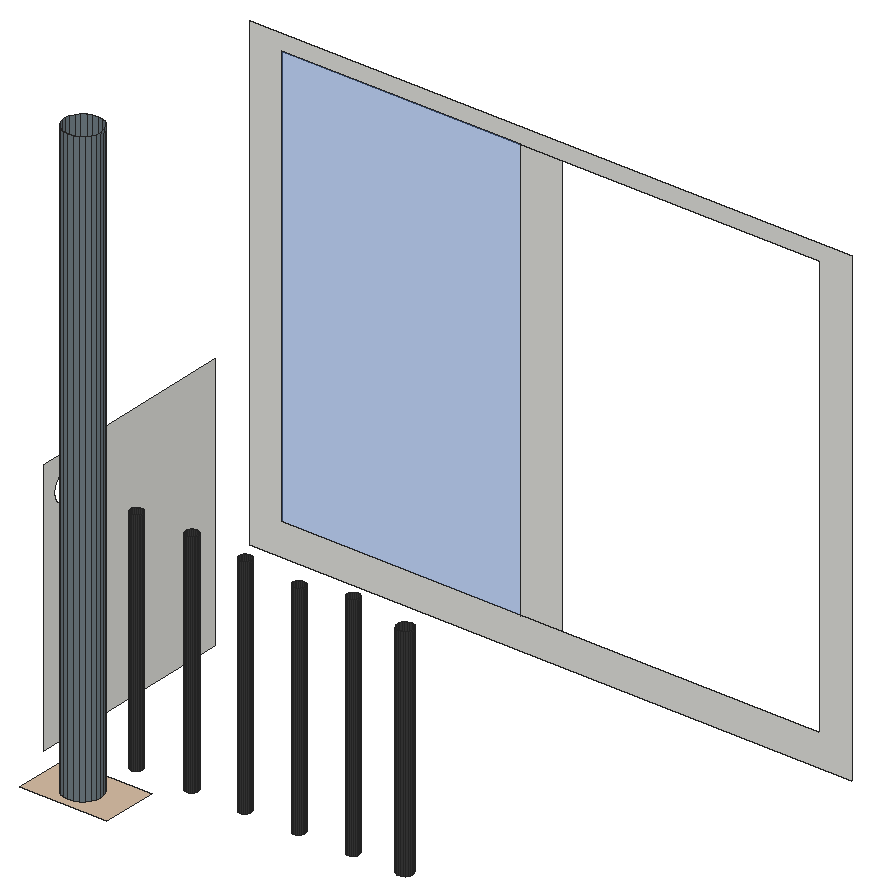
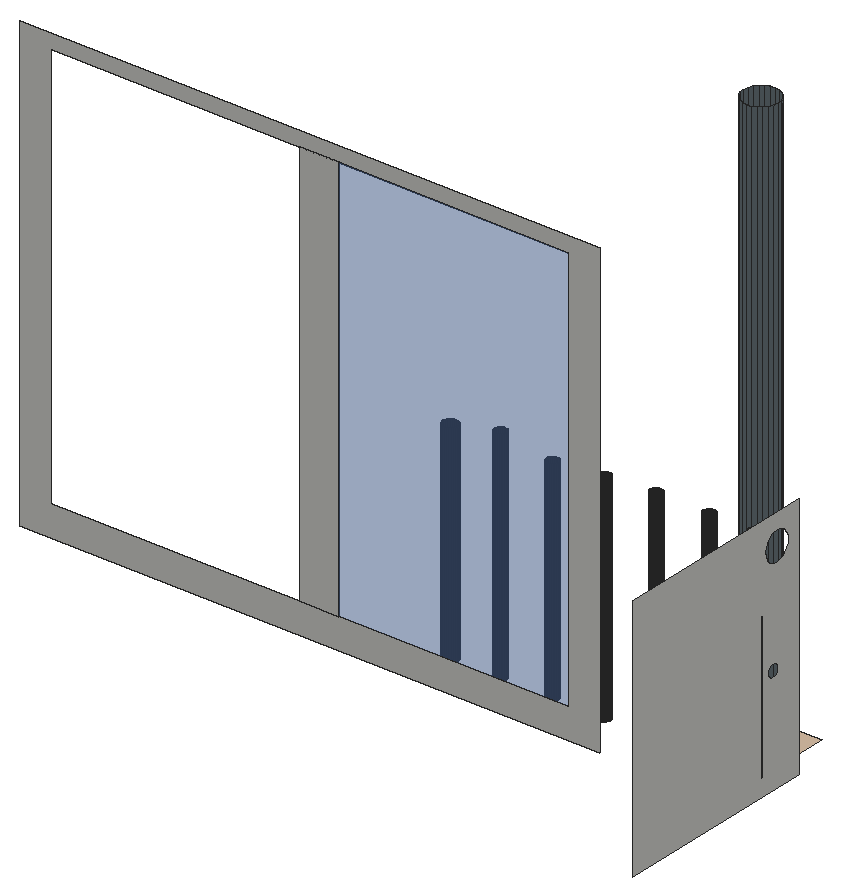
# SketchUp Ruby script. Lengths in inches.
U = 1.inch
M = Sketchup.active_model
def pt(a) = Geom::Point3d.new(a.map { |v| v * U })
def face(e, loops, mat)
  f = e.add_face(loops[0].map { |a| pt(a) })
  loops[1..].each { |l| e.add_face(l.map { |a| pt(a) }).erase! }
  f.material = f.back_material = mat if mat
  f
end
# faces: each face lists its corners as indices into pts; further lists are holes
def faces(e, pts, list, mat = nil) = list.each { |f| face(e, (f[0].is_a?(Array) ? f : [f]).map { |l| l.map { |i| pts[i] } }, mat) }
# xy, xz, yz: faces in a plane at the given z, y or x. An outline is a flat list of corners, or four numbers for a rectangle; further outlines are holes
def ring(l) = l.size == 4 ? [[l[0], l[1]], [l[2], l[1]], [l[2], l[3]], [l[0], l[3]]] : l.each_slice(2).to_a
def flat(e, list, mat, &to3) = list.each { |f| face(e, (f[0].is_a?(Array) ? f : [f]).map { |l| ring(l).map { |u, v| to3.(u, v) } }, mat) }
def xy(e, z, list, mat = nil) = flat(e, list, mat) { |x, y| [x, y, z] }
def xz(e, y, list, mat = nil) = flat(e, list, mat) { |x, z| [x, y, z] }
def yz(e, x, list, mat = nil) = flat(e, list, mat) { |y, z| [x, y, z] }
def lines(e, pts, list) = list.each { |a, b| e.add_line(pt(pts[a]), pt(pts[b])) }
# prism: a flat outline (further loops are holes) pulled along v
def prism(e, loops, v, mat = nil)
  f = face(e, loops, mat); d = Geom::Vector3d.new(v.map { |x| x * U })
  f.pushpull(f.normal.samedirection?(d) ? d.length : -d.length)
end
def box(e, o, s, mat = nil) = prism(e, [[o, [o[0] + s[0], o[1], o[2]], [o[0] + s[0], o[1] + s[1], o[2]], [o[0], o[1] + s[1], o[2]]]], [0, 0, s[2]], mat)
def at(x, y, z, deg = 0) = Geom::Transformation.translation(pt([x, y, z])) * Geom::Transformation.rotation(ORIGIN, Z_AXIS, deg.degrees)
def axes(o, x, y, z) = Geom::Transformation.new([*x, 0, *y, 0, *z, 0, *pt(o).to_a, 1])
def part(name) = M.definitions.add(name)
# library, detail: a bought-in or finely detailed component or shape, given as its bounding box
def library(name, o, s) = part(name).tap { |d| box(d.entities, o, s) }
def detail(e, o, s) = box(e.add_group.entities, o, s)
def put(e, d, t, mat = nil) = e.add_instance(d, t).tap { |i| i.material = mat if mat }
def group(e, t, mat = nil) = e.add_group.tap { |g| g.transformation = t; g.material = mat if mat }.entities
root = M.entities
M.materials.add("[Color M07]").color = [58, 58, 58]
M.materials.add("[Formica Laminate Light]").color = [213, 189, 164]
M.materials.add("[Formica Speckled Grey]").color = [112, 125, 132]
M.materials.add("[Translucent Glass Blue]").color = [85, 126, 201]
M.materials["[Translucent Glass Blue]"].alpha = 0.5
xy(root,273.71,[[54.33,84.29,53.8,84.36,53.3,84.57,52.875,84.89,52.55,85.32,52.34,85.82,52.27,86.35,52.34,86.89,52.55,87.38,52.875,87.8125,53.3,88.14,53.8,88.35,54.33,88.42,54.87,88.35,55.37,88.14,55.79,87.8125,56.12,87.38,56.33,86.89,56.4,86.35,56.33,85.82,56.12,85.32,55.79,84.89,55.37,84.57,54.87,84.36],[85.8,91.86,85.57,91.89,85.36,91.97,85.18,92.11,85.04,92.29,84.95,92.5,84.92,92.73,84.95,92.96,85.04,93.17,85.18,93.35,85.36,93.49,85.57,93.58,85.8,93.61,86.02,93.58,86.24,93.49,86.42,93.35,86.56,93.17,86.64,92.96,86.67,92.73,86.64,92.5,86.56,92.29,86.42,92.11,86.24,91.97,86.02,91.89],[50.09,91.87,49.91,91.89,49.75,91.96,49.61,92.07,49.5,92.21,49.43,92.38,49.4,92.56,49.43,92.73,49.5,92.9,49.61,93.04,49.75,93.15,49.91,93.22,50.09,93.24,50.27,93.22,50.4375,93.15,50.58,93.04,50.6875,92.9,50.76,92.73,50.78,92.56,50.76,92.38,50.6875,92.21,50.58,92.07,50.4375,91.96,50.27,91.89],[55.47,91.87,55.29,91.89,55.125,91.96,54.98,92.07,54.87,92.21,54.8,92.38,54.78,92.56,54.8,92.73,54.87,92.9,54.98,93.04,55.125,93.15,55.29,93.22,55.47,93.24,55.64,93.22,55.8125,93.15,55.95,93.04,56.0625,92.9,56.13,92.73,56.15,92.56,56.13,92.38,56.0625,92.21,55.95,92.07,55.8125,91.96,55.64,91.89],[61.72,91.87,61.54,91.89,61.375,91.96,61.23,92.07,61.12,92.21,61.05,92.38,61.03,92.56,61.05,92.73,61.12,92.9,61.23,93.04,61.375,93.15,61.54,93.22,61.72,93.24,61.89,93.22,62.0625,93.15,62.2,93.04,62.3125,92.9,62.38,92.73,62.4,92.56,62.38,92.38,62.3125,92.21,62.2,92.07,62.0625,91.96,61.89,91.89],
  [67.78,91.87,67.6,91.89,67.4375,91.96,67.29,92.07,67.18,92.21,67.12,92.38,67.09,92.56,67.12,92.73,67.18,92.9,67.29,93.04,67.4375,93.15,67.6,93.22,67.78,93.24,67.96,93.22,68.125,93.15,68.27,93.04,68.375,92.9,68.44,92.73,68.47,92.56,68.44,92.38,68.375,92.21,68.27,92.07,68.125,91.96,67.96,91.89],[73.9,91.87,73.73,91.89,73.5625,91.96,73.42,92.07,73.31,92.21,73.24,92.38,73.22,92.56,73.24,92.73,73.31,92.9,73.42,93.04,73.5625,93.15,73.73,93.22,73.9,93.24,74.08,93.22,74.25,93.15,74.39,93.04,74.5,92.9,74.57,92.73,74.59,92.56,74.57,92.38,74.5,92.21,74.39,92.07,74.25,91.96,74.08,91.89],[80.03,91.87,79.85,91.89,79.6875,91.96,79.54,92.07,79.43,92.21,79.37,92.38,79.34,92.56,79.37,92.73,79.43,92.9,79.54,93.04,79.6875,93.15,79.85,93.22,80.03,93.24,80.21,93.22,80.375,93.15,80.52,93.04,80.625,92.9,80.69,92.73,80.72,92.56,80.69,92.38,80.625,92.21,80.52,92.07,80.375,91.96,80.21,91.89]])
xy(root,273.71,[[[49.6,83.35,59.49,89.73],[54.33,84.29,53.8,84.36,53.3,84.57,52.875,84.89,52.55,85.32,52.34,85.82,52.27,86.35,52.34,86.89,52.55,87.38,52.875,87.8125,53.3,88.14,53.8,88.35,54.33,88.42,54.87,88.35,55.37,88.14,55.79,87.8125,56.12,87.38,56.33,86.89,56.4,86.35,56.33,85.82,56.12,85.32,55.79,84.89,55.37,84.57,54.87,84.36]]],"[Formica Laminate Light]")
xz(root,114.1,[[[51.12,285.36,119.37,338.67],[54.72,288.95,115.77,336.88]],[81.82,288.95,86.49,336.88]])
xz(root,114.1,[[54.72,288.95,81.82,336.88]],"[Translucent Glass Blue]")
yz(root,47.16,[[[89.73,273.71,114.1,302.83],[92.96,297.54,92.51,297.6,92.09,297.77,91.73,298.05,91.45,298.41,91.27,298.84,91.21,299.29,91.27,299.74,91.45,300.16,91.73,300.53,92.09,300.8,92.51,300.98,92.96,301.04,93.42,300.98,93.84,300.8,94.2,300.53,94.48,300.16,94.65,299.74,94.71,299.29,94.65,298.84,94.48,298.41,94.2,298.05,93.84,297.77,93.42,297.6],[93.52,285.62,93.33,285.64,93.15,285.72,92.99,285.84,92.875,285.99,92.8,286.17,92.77,286.37,92.8,286.5625,92.875,286.74,92.99,286.9,93.15,287.02,93.33,287.09,93.52,287.12,93.72,287.09,93.9,287.02,94.05,286.9,94.17,286.74,94.25,286.5625,94.27,286.37,94.25,286.17,94.17,285.99,94.05,285.84,93.9,285.72,93.72,285.64]]])
p = [[53.8,84.36,273.71],[54.33,84.29,273.71],[54.33,84.29,341.31],[53.8,84.36,341.31],[54.87,84.36,273.71],[54.87,84.36,341.31],
  [53.3,84.57,273.71],[53.3,84.57,341.31],[55.37,84.57,273.71],[55.37,84.57,341.31],[52.875,84.89,273.71],[52.875,84.89,341.31],
  [55.79,84.89,273.71],[55.79,84.89,341.31],[52.55,85.32,273.71],[52.55,85.32,341.31],[56.12,85.32,273.71],[56.12,85.32,341.31],
  [52.34,85.82,273.71],[52.34,85.82,341.31],[56.33,85.82,273.71],[56.33,85.82,341.31],[52.27,86.35,273.71],[52.27,86.35,341.31],
  [56.4,86.35,273.71],[56.4,86.35,341.31],[52.34,86.89,273.71],[52.34,86.89,341.31],[56.33,86.89,273.71],[56.33,86.89,341.31],
  [52.55,87.38,273.71],[52.55,87.38,341.31],[56.12,87.38,273.71],[56.12,87.38,341.31],[52.875,87.8125,273.71],[52.875,87.8125,341.31],
  [55.79,87.8125,273.71],[55.79,87.8125,341.31],[53.3,88.14,273.71],[53.3,88.14,341.31],[55.37,88.14,273.71],[55.37,88.14,341.31],
  [53.8,88.35,273.71],[53.8,88.35,341.31],[54.87,88.35,273.71],[54.87,88.35,341.31],[54.33,88.42,273.71],[54.33,88.42,341.31],
  [49.75,91.96,273.71],[49.91,91.89,273.71],[49.91,91.89,299.71],[49.75,91.96,299.71],[50.09,91.87,273.71],[50.09,91.87,299.71],
  [50.27,91.89,273.71],[50.27,91.89,299.71],[50.4375,91.96,273.71],[50.4375,91.96,299.71],[55.125,91.96,273.71],[55.29,91.89,273.71],
  [55.29,91.89,299.74],[55.125,91.96,299.74],[55.47,91.87,273.71],[55.47,91.87,299.74],[55.64,91.89,273.71],[55.64,91.89,299.74],
  [55.8125,91.96,273.71],[55.8125,91.96,299.74],[61.375,91.96,273.71],[61.54,91.89,273.71],[61.54,91.89,299.74],[61.375,91.96,299.74],
  [61.72,91.87,273.71],[61.72,91.87,299.74],[61.89,91.89,273.71],[61.89,91.89,299.74],[62.0625,91.96,273.71],[62.0625,91.96,299.74],
  [67.4375,91.96,273.71],[67.6,91.89,273.71],[67.6,91.89,299.33],[67.4375,91.96,299.33],[67.78,91.87,273.71],[67.78,91.87,299.33],
  [67.96,91.89,273.71],[67.96,91.89,299.33],[68.125,91.96,273.71],[68.125,91.96,299.33],[73.5625,91.96,273.71],[73.73,91.89,273.71],
  [73.73,91.89,298.77],[73.5625,91.96,298.77],[73.9,91.87,273.71],[73.9,91.87,298.77],[74.08,91.89,273.71],[74.08,91.89,298.77],
  [74.25,91.96,273.71],[74.25,91.96,298.77],[79.6875,91.96,273.71],[79.85,91.89,273.71],[79.85,91.89,299.74],[79.6875,91.96,299.74],
  [80.03,91.87,273.71],[80.03,91.87,299.74],[80.21,91.89,273.71],[80.21,91.89,299.74],[80.375,91.96,273.71],[80.375,91.96,299.74],
  [85.36,91.97,273.71],[85.57,91.89,273.71],[85.57,91.89,298.58],[85.36,91.97,298.58],[85.8,91.86,273.71],[85.8,91.86,298.58],
  [86.02,91.89,273.71],[86.02,91.89,298.58],[86.24,91.97,273.71],[86.24,91.97,298.58],[49.61,92.07,273.71],[49.61,92.07,299.71],
  [50.58,92.07,273.71],[50.58,92.07,299.71],[54.98,92.07,273.71],[54.98,92.07,299.74],[55.95,92.07,273.71],[55.95,92.07,299.74],
  [61.23,92.07,273.71],[61.23,92.07,299.74],[62.2,92.07,273.71],[62.2,92.07,299.74],[67.29,92.07,273.71],[67.29,92.07,299.33],
  [68.27,92.07,273.71],[68.27,92.07,299.33],[73.42,92.07,273.71],[73.42,92.07,298.77],[74.39,92.07,273.71],[74.39,92.07,298.77],
  [79.54,92.07,273.71],[79.54,92.07,299.74],[80.52,92.07,273.71],[80.52,92.07,299.74],[85.18,92.11,273.71],[85.18,92.11,298.58],
  [86.42,92.11,273.71],[86.42,92.11,298.58],[49.5,92.21,273.71],[49.5,92.21,299.71],[50.6875,92.21,273.71],[50.6875,92.21,299.71],
  [54.87,92.21,273.71],[54.87,92.21,299.74],[56.0625,92.21,273.71],[56.0625,92.21,299.74],[61.12,92.21,273.71],[61.12,92.21,299.74],
  [62.3125,92.21,273.71],[62.3125,92.21,299.74],[67.18,92.21,273.71],[67.18,92.21,299.33],[68.375,92.21,273.71],[68.375,92.21,299.33],
  [73.31,92.21,273.71],[73.31,92.21,298.77],[74.5,92.21,273.71],[74.5,92.21,298.77],[79.43,92.21,273.71],[79.43,92.21,299.74],
  [80.625,92.21,273.71],[80.625,92.21,299.74],[85.04,92.29,273.71],[85.04,92.29,298.58],[86.56,92.29,273.71],[86.56,92.29,298.58],
  [49.43,92.38,273.71],[49.43,92.38,299.71],[50.76,92.38,273.71],[50.76,92.38,299.71],[54.8,92.38,273.71],[54.8,92.38,299.74],
  [56.13,92.38,273.71],[56.13,92.38,299.74],[61.05,92.38,273.71],[61.05,92.38,299.74],[62.38,92.38,273.71],[62.38,92.38,299.74],
  [67.12,92.38,273.71],[67.12,92.38,299.33],[68.44,92.38,273.71],[68.44,92.38,299.33],[73.24,92.38,273.71],[73.24,92.38,298.77],
  [74.57,92.38,273.71],[74.57,92.38,298.77],[79.37,92.38,273.71],[79.37,92.38,299.74],[80.69,92.38,273.71],[80.69,92.38,299.74],
  [84.95,92.5,273.71],[84.95,92.5,298.58],[86.64,92.5,273.71],[86.64,92.5,298.58],[49.4,92.56,273.71],[49.4,92.56,299.71],
  [50.78,92.56,273.71],[50.78,92.56,299.71],[54.78,92.56,273.71],[54.78,92.56,299.74],[56.15,92.56,273.71],[56.15,92.56,299.74],
  [61.03,92.56,273.71],[61.03,92.56,299.74],[62.4,92.56,273.71],[62.4,92.56,299.74],[67.09,92.56,273.71],[67.09,92.56,299.33],
  [68.47,92.56,273.71],[68.47,92.56,299.33],[73.22,92.56,273.71],[73.22,92.56,298.77],[74.59,92.56,273.71],[74.59,92.56,298.77],
  [79.34,92.56,273.71],[79.34,92.56,299.74],[80.72,92.56,273.71],[80.72,92.56,299.74],[84.92,92.73,273.71],[84.92,92.73,298.58],
  [86.67,92.73,273.71],[86.67,92.73,298.58],[49.43,92.73,273.71],[49.43,92.73,299.71],[50.76,92.73,273.71],[50.76,92.73,299.71],
  [54.8,92.73,273.71],[54.8,92.73,299.74],[56.13,92.73,273.71],[56.13,92.73,299.74],[61.05,92.73,273.71],[61.05,92.73,299.74],
  [62.38,92.73,273.71],[62.38,92.73,299.74],[67.12,92.73,273.71],[67.12,92.73,299.33],[68.44,92.73,273.71],[68.44,92.73,299.33],
  [73.24,92.73,273.71],[73.24,92.73,298.77],[74.57,92.73,273.71],[74.57,92.73,298.77],[79.37,92.73,273.71],[79.37,92.73,299.74],
  [80.69,92.73,273.71],[80.69,92.73,299.74],[49.5,92.9,273.71],[49.5,92.9,299.71],[50.6875,92.9,273.71],[50.6875,92.9,299.71],
  [54.87,92.9,273.71],[54.87,92.9,299.74],[56.0625,92.9,273.71],[56.0625,92.9,299.74],[61.12,92.9,273.71],[61.12,92.9,299.74],
  [62.3125,92.9,273.71],[62.3125,92.9,299.74],[67.18,92.9,273.71],[67.18,92.9,299.33],[68.375,92.9,273.71],[68.375,92.9,299.33],
  [73.31,92.9,273.71],[73.31,92.9,298.77],[74.5,92.9,273.71],[74.5,92.9,298.77],[79.43,92.9,273.71],[79.43,92.9,299.74],
  [80.625,92.9,273.71],[80.625,92.9,299.74],[84.95,92.96,273.71],[84.95,92.96,298.58],[86.64,92.96,273.71],[86.64,92.96,298.58],
  [49.61,93.04,273.71],[49.61,93.04,299.71],[50.58,93.04,273.71],[50.58,93.04,299.71],[54.98,93.04,273.71],[54.98,93.04,299.74],
  [55.95,93.04,273.71],[55.95,93.04,299.74],[61.23,93.04,273.71],[61.23,93.04,299.74],[62.2,93.04,273.71],[62.2,93.04,299.74],
  [67.29,93.04,273.71],[67.29,93.04,299.33],[68.27,93.04,273.71],[68.27,93.04,299.33],[73.42,93.04,273.71],[73.42,93.04,298.77],
  [74.39,93.04,273.71],[74.39,93.04,298.77],[79.54,93.04,273.71],[79.54,93.04,299.74],[80.52,93.04,273.71],[80.52,93.04,299.74],
  [49.75,93.15,273.71],[49.75,93.15,299.71],[50.4375,93.15,273.71],[50.4375,93.15,299.71],[55.125,93.15,273.71],[55.125,93.15,299.74],
  [55.8125,93.15,273.71],[55.8125,93.15,299.74],[61.375,93.15,273.71],[61.375,93.15,299.74],[62.0625,93.15,273.71],[62.0625,93.15,299.74],
  [67.4375,93.15,273.71],[67.4375,93.15,299.33],[68.125,93.15,273.71],[68.125,93.15,299.33],[73.5625,93.15,273.71],[73.5625,93.15,298.77],
  [74.25,93.15,273.71],[74.25,93.15,298.77],[79.6875,93.15,273.71],[79.6875,93.15,299.74],[80.375,93.15,273.71],[80.375,93.15,299.74],
  [85.04,93.17,273.71],[85.04,93.17,298.58],[86.56,93.17,273.71],[86.56,93.17,298.58],[49.91,93.22,273.71],[49.91,93.22,299.71],
  [50.09,93.24,273.71],[50.09,93.24,299.71],[50.27,93.22,273.71],[50.27,93.22,299.71],[55.29,93.22,273.71],[55.29,93.22,299.74],
  [55.47,93.24,273.71],[55.47,93.24,299.74],[55.64,93.22,273.71],[55.64,93.22,299.74],[61.54,93.22,273.71],[61.54,93.22,299.74],
  [61.72,93.24,273.71],[61.72,93.24,299.74],[61.89,93.22,273.71],[61.89,93.22,299.74],[67.6,93.22,273.71],[67.6,93.22,299.33],
  [67.78,93.24,273.71],[67.78,93.24,299.33],[67.96,93.22,273.71],[67.96,93.22,299.33],[73.73,93.22,273.71],[73.73,93.22,298.77],
  [73.9,93.24,273.71],[73.9,93.24,298.77],[74.08,93.22,273.71],[74.08,93.22,298.77],[79.85,93.22,273.71],[79.85,93.22,299.74],
  [80.03,93.24,273.71],[80.03,93.24,299.74],[80.21,93.22,273.71],[80.21,93.22,299.74],[85.18,93.35,273.71],[85.18,93.35,298.58],
  [86.42,93.35,273.71],[86.42,93.35,298.58],[85.36,93.49,273.71],[85.36,93.49,298.58],[86.24,93.49,273.71],[86.24,93.49,298.58],
  [85.57,93.58,273.71],[85.57,93.58,298.58],[86.02,93.58,273.71],[86.02,93.58,298.58],[85.8,93.61,273.71],[85.8,93.61,298.58]]
faces(root,p,[[0,1,2,3],[1,4,5,2],[6,0,3,7],[4,8,9,5],[10,6,7,11],[8,12,13,9],[14,10,11,15],[12,16,17,13],
  [18,14,15,19],[16,20,21,17],[22,18,19,23],[20,24,25,21],[26,22,23,27],[24,28,29,25],[30,26,27,31],[28,32,33,29],
  [34,30,31,35],[32,36,37,33],[38,34,35,39],[36,40,41,37],[42,38,39,43],[40,44,45,41],[46,42,43,47],[44,46,47,45]],"[Formica Speckled Grey]")
faces(root,p,[[48,49,50,51],[49,52,53,50],[52,54,55,53],[54,56,57,55],[58,59,60,61],[59,62,63,60],[62,64,65,63],[64,66,67,65],
  [68,69,70,71],[69,72,73,70],[72,74,75,73],[74,76,77,75],[78,79,80,81],[79,82,83,80],[82,84,85,83],[84,86,87,85],
  [88,89,90,91],[89,92,93,90],[92,94,95,93],[94,96,97,95],[98,99,100,101],[99,102,103,100],[102,104,105,103],[104,106,107,105],
  [108,109,110,111],[109,112,113,110],[112,114,115,113],[114,116,117,115],[118,48,51,119],[56,120,121,57],[122,58,61,123],[66,124,125,67],
  [126,68,71,127],[76,128,129,77],[130,78,81,131],[86,132,133,87],[134,88,91,135],[96,136,137,97],[138,98,101,139],[106,140,141,107],
  [142,108,111,143],[116,144,145,117],[146,118,119,147],[120,148,149,121],[150,122,123,151],[124,152,153,125],[154,126,127,155],[128,156,157,129],
  [158,130,131,159],[132,160,161,133],[162,134,135,163],[136,164,165,137],[166,138,139,167],[140,168,169,141],[170,142,143,171],[144,172,173,145],
  [174,146,147,175],[148,176,177,149],[178,150,151,179],[152,180,181,153],[182,154,155,183],[156,184,185,157],[186,158,159,187],[160,188,189,161],
  [190,162,163,191],[164,192,193,165],[194,166,167,195],[168,196,197,169],[198,170,171,199],[172,200,201,173],[202,174,175,203],[176,204,205,177],
  [206,178,179,207],[180,208,209,181],[210,182,183,211],[184,212,213,185],[214,186,187,215],[188,216,217,189],[218,190,191,219],[192,220,221,193],
  [222,194,195,223],[196,224,225,197],[226,198,199,227],[200,228,229,201],[230,202,203,231],[204,232,233,205],[234,206,207,235],[208,236,237,209],
  [238,210,211,239],[212,240,241,213],[242,214,215,243],[216,244,245,217],[246,218,219,247],[220,248,249,221],[250,222,223,251],[224,252,253,225],
  [254,230,231,255],[232,256,257,233],[258,234,235,259],[236,260,261,237],[262,238,239,263],[240,264,265,241],[266,242,243,267],[244,268,269,245],
  [270,246,247,271],[248,272,273,249],[274,250,251,275],[252,276,277,253],[278,226,227,279],[228,280,281,229],[282,254,255,283],[256,284,285,257],
  [286,258,259,287],[260,288,289,261],[290,262,263,291],[264,292,293,265],[294,266,267,295],[268,296,297,269],[298,270,271,299],[272,300,301,273],
  [302,274,275,303],[276,304,305,277],[306,282,283,307],[284,308,309,285],[310,286,287,311],[288,312,313,289],[314,290,291,315],[292,316,317,293],
  [318,294,295,319],[296,320,321,297],[322,298,299,323],[300,324,325,301],[326,302,303,327],[304,328,329,305],[330,278,279,331],[280,332,333,281],
  [334,306,307,335],[336,334,335,337],[338,336,337,339],[308,338,339,309],[340,310,311,341],[342,340,341,343],[344,342,343,345],[312,344,345,313],
  [346,314,315,347],[348,346,347,349],[350,348,349,351],[316,350,351,317],[352,318,319,353],[354,352,353,355],[356,354,355,357],[320,356,357,321],
  [358,322,323,359],[360,358,359,361],[362,360,361,363],[324,362,363,325],[364,326,327,365],[366,364,365,367],[368,366,367,369],[328,368,369,329],
  [370,330,331,371],[332,372,373,333],[374,370,371,375],[372,376,377,373],[378,374,375,379],[376,380,381,377],[382,378,379,383],[380,382,383,381]],"[Color M07]")
